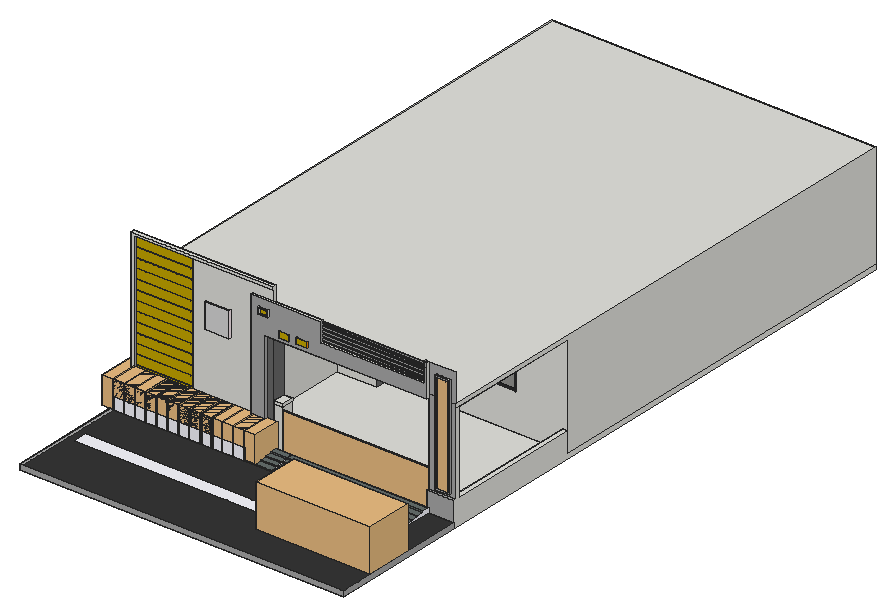
# SketchUp Ruby script. Lengths in inches.
U = 1.inch
M = Sketchup.active_model
def pt(a) = Geom::Point3d.new(a.map { |v| v * U })
def face(e, loops, mat)
  f = e.add_face(loops[0].map { |a| pt(a) })
  loops[1..].each { |l| e.add_face(l.map { |a| pt(a) }).erase! }
  f.material = f.back_material = mat if mat
  f
end
# faces: each face lists its corners as indices into pts; further lists are holes
def faces(e, pts, list, mat = nil) = list.each { |f| face(e, (f[0].is_a?(Array) ? f : [f]).map { |l| l.map { |i| pts[i] } }, mat) }
# xy, xz, yz: faces in a plane at the given z, y or x. An outline is a flat list of corners, or four numbers for a rectangle; further outlines are holes
def ring(l) = l.size == 4 ? [[l[0], l[1]], [l[2], l[1]], [l[2], l[3]], [l[0], l[3]]] : l.each_slice(2).to_a
def flat(e, list, mat, &to3) = list.each { |f| face(e, (f[0].is_a?(Array) ? f : [f]).map { |l| ring(l).map { |u, v| to3.(u, v) } }, mat) }
def xy(e, z, list, mat = nil) = flat(e, list, mat) { |x, y| [x, y, z] }
def xz(e, y, list, mat = nil) = flat(e, list, mat) { |x, z| [x, y, z] }
def yz(e, x, list, mat = nil) = flat(e, list, mat) { |y, z| [x, y, z] }
def lines(e, pts, list) = list.each { |a, b| e.add_line(pt(pts[a]), pt(pts[b])) }
# prism: a flat outline (further loops are holes) pulled along v
def prism(e, loops, v, mat = nil)
  f = face(e, loops, mat); d = Geom::Vector3d.new(v.map { |x| x * U })
  f.pushpull(f.normal.samedirection?(d) ? d.length : -d.length)
end
def box(e, o, s, mat = nil) = prism(e, [[o, [o[0] + s[0], o[1], o[2]], [o[0] + s[0], o[1] + s[1], o[2]], [o[0], o[1] + s[1], o[2]]]], [0, 0, s[2]], mat)
def at(x, y, z, deg = 0) = Geom::Transformation.translation(pt([x, y, z])) * Geom::Transformation.rotation(ORIGIN, Z_AXIS, deg.degrees)
def axes(o, x, y, z) = Geom::Transformation.new([*x, 0, *y, 0, *z, 0, *pt(o).to_a, 1])
def part(name) = M.definitions.add(name)
# library, detail: a bought-in or finely detailed component or shape, given as its bounding box
def library(name, o, s) = part(name).tap { |d| box(d.entities, o, s) }
def detail(e, o, s) = box(e.add_group.entities, o, s)
def put(e, d, t, mat = nil) = e.add_instance(d, t).tap { |i| i.material = mat if mat }
def group(e, t, mat = nil) = e.add_group.tap { |g| g.transformation = t; g.material = mat if mat }.entities
root = M.entities
M.materials.add("Glass_Tinted_Gray").color = [0, 0, 0]
M.materials["Glass_Tinted_Gray"].alpha = 0.125
M.materials.add("Shane").color = [124, 51, 43]
M.materials.add("[0008_LavenderBlush]").color = [255, 240, 245]
M.materials.add("[0019_Crimson]").color = [215, 215, 215]
M.materials.add("[0039_DarkOrange]").color = [255, 140, 0]
M.materials.add("[0046_Gold]").color = [198, 167, 0]
M.materials.add("[0117_GhostWhite]").color = [248, 248, 255]
M.materials.add("[0132_LightGray]").color = [169, 169, 169]
M.materials.add("[0134_DimGray]").color = [105, 105, 105]
M.materials.add("[0135_DarkGray]").color = [81, 81, 81]
M.materials.add("[Mirror 02]").color = [229, 229, 229]
M.materials.add("[Slate Light Tile]").color = [54, 54, 54]
M.materials.add("[Slate]").color = [102, 110, 108]
M.materials.add("[Terrazzo Light Blue]").color = [196, 214, 227]
c1 = part("door 15\#1")
xy(c1.entities,0,[[0,0,0,6,2.34,6,2.34,4,33.41,4,33.41,6,36.21,6,36.21,0,33.4,0,33.4,2,3.22,2,3.22,0]],"Shane")
xy(c1.entities,78.49,[[3.22,0,33.4,2]],"Shane")
xy(c1.entities,78.6875,[[2.34,4,33.41,6]],"Shane")
xy(c1.entities,80.63,[[0,0,36.21,6]],"Shane")
xz(c1.entities,0,[[0,0,3.22,0,3.22,78.49,33.4,78.49,33.4,0,36.21,0,36.21,80.63,0,80.63]],"Shane")
xz(c1.entities,2,[[3.22,0,33.4,78.49]],"Shane")
xz(c1.entities,4,[[2.34,0,33.41,78.6875]],"Shane")
xz(c1.entities,6,[[0,0,0,80.63,36.21,80.63,36.21,0,33.41,0,33.41,78.6875,2.34,78.6875,2.34,0]],"Shane")
yz(c1.entities,0,[[0,0,6,80.63]],"Shane")
yz(c1.entities,2.34,[[4,0,6,78.6875]],"Shane")
yz(c1.entities,3.22,[[0,0,2,78.49]],"Shane")
yz(c1.entities,33.4,[[0,0,2,78.49]],"Shane")
yz(c1.entities,33.41,[[4,0,6,78.6875]],"Shane")
yz(c1.entities,36.21,[[0,0,6,80.63]],"Shane")
c2 = part("PENTEK_RP Fineline 50S_Sliding_DoorCase_E1")
box(c2.entities,[0,0,0],[1.51,3.66,99.27],"[0135_DarkGray]")
c3 = part("PENTEK_RP Fineline 50S_SlidingDooe_Case_E2")
box(c3.entities,[0,0,0],[96.25,3.66,1.51],"[0135_DarkGray]")
c4 = part("pentek_RP Fineline 50S_SlidingDoor_Case")
put(c4.entities,c2,at(97.76,0,0))
put(c4.entities,c3,at(1.51,0,0))
put(c4.entities,c2,at(0,0,0))
put(c4.entities,c3,at(1.51,0,97.76))
c5 = part("PENTEK_RP Fineline 50S_SlidingDoor_GlazingBead_2")
box(c5.entities,[0,0,0],[0.56,0.59,94.39],"[0135_DarkGray]")
c6 = part("PENTEK_RP Fineline 50S_SlidingDoor_Glass")
box(c6.entities,[0,0,0],[46.58,0.16,94.39],"Glass_Tinted_Gray")
c7 = part("PENTEK_RP Fineline 50S_SlidingDoor_GlazingBead")
box(c7.entities,[0,0,0],[45.47,0.59,0.56],"[0135_DarkGray]")
c8 = part("PENTEK_RP Fineline 50S_SlidingDoor_Leaf_E1")
xy(c8.entities,0,[[0,0,0.93,1.97],[0.93,1.57,1.49,1.97]],"[0135_DarkGray]")
xy(c8.entities,96.25,[[0,0,0.93,0,0.93,1.57,1.49,1.57,1.49,1.97,0,1.97]],"[0135_DarkGray]")
xz(c8.entities,0,[[0,0,0.93,96.25]],"[0135_DarkGray]")
xz(c8.entities,1.57,[[0.93,0,1.49,95.32],[0.93,95.32,1.49,96.25]],"[0135_DarkGray]")
xz(c8.entities,1.97,[[0,0,1.49,96.25]],"[0135_DarkGray]")
yz(c8.entities,0,[[0,0,1.97,96.25]],"[0135_DarkGray]")
yz(c8.entities,0.93,[[0,0,1.57,0.93],[0,0.93,1.57,95.32],[0,95.32,1.57,96.25]],"[0135_DarkGray]")
yz(c8.entities,1.49,[[1.57,0,1.97,95.32],[1.57,95.32,1.97,96.25]],"[0135_DarkGray]")
c9 = part("PENTEK_RP Fineline 50S_SlidingDoor_Leaf_E2")
xy(c9.entities,0,[[0,0,0,1.57,0.56,1.57,0.56,1.97,46.02,1.97,46.02,1.57,46.58,1.57,46.58,0]],"[0135_DarkGray]")
xy(c9.entities,0.93,[[0,0,46.58,1.57]],"[0135_DarkGray]")
xy(c9.entities,1.49,[[0.56,1.57,46.02,1.97]],"[0135_DarkGray]")
xz(c9.entities,0,[[0,0,46.58,0.93]],"[0135_DarkGray]")
xz(c9.entities,1.57,[[0,0,0.56,0.93],[46.02,0,46.58,0.93],[0.56,0.93,46.02,1.49]],"[0135_DarkGray]")
xz(c9.entities,1.97,[[0.56,0,46.02,1.49]],"[0135_DarkGray]")
yz(c9.entities,0,[[0,0,1.57,0.93]],"[0135_DarkGray]")
yz(c9.entities,0.56,[[1.57,0,1.97,0.93],[1.57,0.93,1.97,1.49]],"[0135_DarkGray]")
yz(c9.entities,46.02,[[1.57,0,1.97,0.93],[1.57,0.93,1.97,1.49]],"[0135_DarkGray]")
yz(c9.entities,46.58,[[0,0,1.57,0.93]],"[0135_DarkGray]")
c10 = part("PENTEK_RP Fineline S_SlidingDoor_Leaf1")
put(c10.entities,c5,at(0.93,0,0.93))
put(c10.entities,c5,at(46.96,0,0.93))
put(c10.entities,c6,at(1.49,1.42,0.93))
put(c10.entities,c7,at(1.49,0,0.93))
put(c10.entities,c6,at(1.49,0.59,0.93),"[Terrazzo Light Blue]")
put(c10.entities,c8,at(0,0,0))
put(c10.entities,c8,axes([48.44,0,0],[-1,0,0],[0,1,0],[0,0,1]))
put(c10.entities,c9,axes([0.93,0,96.25],[1,0,0],[0,1,0],[0,0,-1]))
put(c10.entities,c9,at(0.93,0,0))
put(c10.entities,c7,at(1.49,0,94.77))
c11 = part("PENTEK_RP Fineline 50S_SlidingDoor_Leaf2")
put(c11.entities,c6,at(1.49,1.42,0.93))
put(c11.entities,c7,at(1.49,0,94.77))
put(c11.entities,c5,at(46.96,0,0.93))
put(c11.entities,c6,at(1.49,0.59,0.93),"[Mirror 02]")
put(c11.entities,c5,at(0.93,0,0.93))
put(c11.entities,c8,at(0,0,0))
put(c11.entities,c8,axes([48.44,0,0],[-1,0,0],[0,1,0],[0,0,1]))
put(c11.entities,c7,at(1.49,0,0.93))
put(c11.entities,c9,axes([0.93,0,96.25],[1,0,0],[0,1,0],[0,0,-1]))
put(c11.entities,c9,at(0.93,0,0))
c12 = part("PENTEK - Slimmest Steel Sliding Door / Window\#1")
put(c12.entities,c4,at(0,-1.88,-0.09))
put(c12.entities,c10,at(1.51,-2.27,1.42))
put(c12.entities,c11,at(49.32,-0.3,1.42))
c13 = library("new block.dwg",[0,0,0],[18.5,26.77,0.5])
c14 = library("Modern Gate 1",[0,0,0],[118.11,1.97,78.74])
c15 = library("Toyota Hilux",[0,0,0],[260.73,623.23,228.58])
c16 = part("car")
put(c16.entities,c15,axes([0,623.33,0.01],[1,0,0],[0,-1,0],[0,0,1]))
c17 = library("Palm",[82.2,-9.29,-2.36],[51.18,55.77,65.42])
c18 = library("Pinch Pot",[-27.95,-27.95,0],[55.9,55.9,47.42])
c19 = part("Potted palm")
put(c19.entities,c17,axes([3796.42,-10488.37,43.97],[0,116.51338,0],[-116.51338,0,0],[0,0,116.51338]))
put(c19.entities,c18,axes([1647.67,1801.1875,0],[0,30.58476,0],[-30.58476,0,0],[0,0,45.1095]))
c20 = library("Dome Light",[-12,-12,0],[24,24,12])
xy(root,-6,[[0,158.125,369.9375,761.125]])
xy(root,-6,[[0,0,369.9375,158.125]],"[0132_LightGray]")
xy(root,0,[[161.72,158.125,338.91,158.125,338.91,164.5,363.9375,164.5,363.9375,321.3125,217.72,321.3125,217.72,365,170.41,365,170.41,321.3125,161.72,321.3125,161.72,307.89,116.03,307.89,116.03,174.55,161.72,174.55,161.72,174.375,171.53,174.375,171.53,161.125,161.72,161.125],[0,159.125,4,159.125,4,160.625,68.79,160.625,68.79,161.125,161.72,161.125,161.72,174.55,116.03,174.55,116.03,307.89,161.72,307.89,161.72,321.3125,170.41,321.3125,170.41,365,217.72,365,217.72,321.3125,369.9375,321.3125,369.9375,761.125,0,761.125]])
xy(root,0,[[12.52,63.38,351.27,78.51],[184.6875,129.125,340.6875,158.125],[6.76,131.88,151.49,155.37]],"[0117_GhostWhite]")
xy(root,0,[[0,0,4,129.125],[0,129.125,4,158.125],[154.25,129.125,184.6875,158.125],[0,158.125,4,159.125],[4,158.125,68.79,160.625],
  [68.79,158.125,137.31,161.125],[137.31,158.125,153.78,161.125],[153.78,158.125,161.72,161.125]],"[0132_LightGray]")
xy(root,0,[[[4,0,369.9375,0,369.9375,158.125,340.6875,158.125,340.6875,129.125,4,129.125],[12.52,63.38,351.27,78.51]]],"[Slate Light Tile]")
xy(root,1.25,[[154.25,129.125,184.6875,136.375],[184.6875,129.125,340.6875,136.375]],"[Slate]")
xy(root,2.375,[[154.25,136.375,184.6875,143.625],[184.6875,136.375,340.6875,143.625]],"[Slate]")
xy(root,3.5,[[154.25,143.625,184.6875,150.875],[184.6875,143.625,340.6875,150.875]],"[Slate]")
xy(root,4.875,[[154.25,150.875,184.6875,158.125],[184.6875,150.875,340.6875,158.125]],"[Slate]")
xy(root,10.38,[[4,160.625,68.79,161.125]])
xy(root,10.98,[[4,160.625,68.79,161.125]])
xy(root,13.4375,[[[4,129.125,154.25,158.125],[6.76,131.88,151.49,155.37]]],"[0117_GhostWhite]")
xy(root,21.37,[[4,160.625,68.79,161.125]])
xy(root,21.97,[[4,160.625,68.79,161.125]])
xy(root,22.8125,[[363.9375,164.5,369.9375,321.3125]])
xy(root,22.8125,[[338.91,158.125,369.9375,161.125]],"[0132_LightGray]")
xy(root,25.96,[[347.38,158.75,364.45,161.125]])
xy(root,28.16,[[349.58,158.75,362.25,161.125]])
xy(root,32.35,[[4,160.625,68.79,161.125]])
xy(root,32.95,[[4,160.625,68.79,161.125]])
xy(root,41.52,[[244.46,321.3125,309.58,347.625]])
xy(root,43.33,[[4,160.625,68.79,161.125]])
xy(root,43.93,[[4,160.625,68.79,161.125]])
xy(root,48,[[161.72,160.625,172.03,161.125],[161.72,161.125,171.53,174.375],[171.53,161.125,172.03,174.55],[161.72,174.375,171.53,174.55]])
xy(root,51,[[161.72,160.625,172.03,174.55]])
xy(root,54.32,[[4,160.625,68.79,161.125]])
xy(root,54.92,[[4,160.625,68.79,161.125]])
xy(root,65.3,[[4,160.625,68.79,161.125]])
xy(root,65.9,[[4,160.625,68.79,161.125]])
xy(root,76.28,[[4,160.625,68.79,161.125]])
xy(root,76.88,[[4,160.625,68.79,161.125]])
xy(root,87.27,[[4,160.625,68.79,161.125]])
xy(root,87.87,[[4,160.625,68.79,161.125]])
xy(root,93.58,[[244.46,321.3125,309.58,347.625]])
xy(root,94.375,[[170.41,321.3125,217.72,365]])
xy(root,97.96,[[84.13,158.5625,111.94,161.125]],"[0008_LavenderBlush]")
xy(root,98.25,[[4,160.625,68.79,161.125]])
xy(root,98.85,[[4,160.625,68.79,161.125]])
xy(root,102.58,[[116.03,174.55,161.72,307.89]])
xy(root,109.23,[[4,160.625,68.79,161.125]])
xy(root,109.83,[[4,160.625,68.79,161.125]])
xy(root,116,[[161.72,161.125,161.72,321.3125,271.17,321.3125,367.86,164.5,338.91,164.5,338.91,161.125],[369.9375,161.125,367.86,164.5,369.9375,164.5],[367.86,164.5,271.17,321.3125,369.9375,321.3125,369.9375,164.5]])
xy(root,116,[[153.78,158.125,338.91,161.125]],"[0132_LightGray]")
xy(root,119.85,[[170.43,157.43,181.45,158.125]],"[0039_DarkOrange]")
xy(root,120,[[161.72,161.125,369.9375,161.125,369.9375,761.125,0,761.125,0,163.25,161.72,163.25]])
xy(root,120.17,[[189.76,157.43,202.51,158.125]],"[0039_DarkOrange]")
xy(root,120.22,[[4,160.625,68.79,161.125]])
xy(root,120.82,[[4,160.625,68.79,161.125]])
xy(root,125.77,[[84.13,158.5625,111.94,161.125]],"[0008_LavenderBlush]")
xy(root,126.67,[[170.43,157.43,181.45,158.125]],"[0039_DarkOrange]")
xy(root,126.74,[[189.76,157.43,202.51,158.125]],"[0039_DarkOrange]")
xy(root,131.0625,[[217.73,158.125,335.04,161.125]])
xy(root,131.2,[[4,160.625,68.79,161.125]])
xy(root,131.8,[[4,160.625,68.79,161.125]])
xy(root,133.74,[[217.73,158.86,335.73,160.42]])
xy(root,135.3,[[217.73,158.86,335.73,160.42]],"[0132_LightGray]")
xy(root,136.46,[[146.93,156.6875,158.46,158.125]])
xy(root,137.27,[[147.74,156.6875,157.65,158.125]])
xy(root,137.93,[[217.73,158.86,336.85,160.42]])
xy(root,139.49,[[217.73,158.86,336.85,160.42]],"[0132_LightGray]")
xy(root,141.33,[[349.58,158.75,362.25,161.125]])
xy(root,142.11,[[217.73,158.86,337.16,160.42]])
xy(root,142.18,[[4,160.625,68.79,161.125]])
xy(root,142.78,[[147.74,156.6875,157.65,158.125],[4,160.625,68.79,161.125]])
xy(root,143.53,[[347.38,158.75,364.45,161.125]])
xy(root,143.59,[[146.93,156.6875,158.46,158.125]])
xy(root,143.68,[[217.73,158.86,337.16,160.42]],"[0132_LightGray]")
xy(root,146.3,[[217.73,158.86,336.54,160.42]])
xy(root,147.86,[[217.73,158.86,336.54,160.42]])
xy(root,150.49,[[217.73,158.86,338.66,160.42]])
xy(root,152.05,[[217.73,158.86,338.66,160.42]])
xy(root,152.8125,[[137.31,158.125,217.73,161.125],[335.04,158.125,338.91,161.125]])
xy(root,153.17,[[4,160.625,68.79,161.125]])
xy(root,153.77,[[4,160.625,68.79,161.125]])
xy(root,164.75,[[4,159.125,4,160.625,68.79,160.625,68.79,161.125,161.72,161.125,161.72,159.125]])
xy(root,168,[[0,159.125,161.72,163.25]])
xz(root,0,[[0,-6,369.9375,0]],"[0132_LightGray]")
xz(root,129.125,[[4,0,154.25,13.4375]],"[0117_GhostWhite]")
xz(root,129.125,[[154.25,0,184.6875,1.25]],"[0132_LightGray]")
xz(root,129.125,[[184.6875,0,340.6875,1.25]],"[Slate]")
xz(root,131.88,[[6.76,0,151.49,13.4375]],"[0117_GhostWhite]")
xz(root,136.375,[[154.25,1.25,184.6875,2.375],[184.6875,1.25,340.6875,2.375]],"[Slate]")
xz(root,143.625,[[154.25,2.375,184.6875,3.5],[184.6875,2.375,340.6875,3.5]],"[Slate]")
xz(root,150.875,[[154.25,3.5,184.6875,4.875],[184.6875,3.5,340.6875,4.875]],"[Slate]")
xz(root,155.37,[[6.76,0,151.49,13.4375]],"[0117_GhostWhite]")
xz(root,156.6875,[[[146.93,136.46,158.46,143.59],[147.74,137.27,157.65,142.78]]])
xz(root,157.43,[[170.43,119.85,181.45,126.67],[189.76,120.17,202.51,126.74]],"[0046_Gold]")
xz(root,158.125,[[147.74,137.27,157.65,142.78]],"[0046_Gold]")
xz(root,158.125,[[184.6875,0,338.91,4.875]],"[0117_GhostWhite]")
xz(root,158.125,[[0,-6,369.9375,0],[4,0,68.79,13.4375],[68.79,0,137.31,13.4375],[137.31,0,153.78,13.4375],[153.78,0,154.25,13.4375],
  [154.25,0,184.6875,4.875],[338.91,0,340.6875,4.875],[340.6875,0,369.9375,0,369.9375,22.8125,338.91,22.8125,338.91,4.875,340.6875,4.875],[[137.31,13.4375,153.78,13.4375,153.78,116,338.91,116,338.91,152.8125,335.04,152.8125,335.04,131.0625,217.73,131.0625,217.73,152.8125,137.31,152.8125],[189.76,120.17,202.51,126.74],[146.93,136.46,158.46,143.59],[170.43,119.85,181.45,126.67]]],"[0132_LightGray]")
xz(root,158.5625,[[84.13,97.96,111.94,125.77]],"[0019_Crimson]")
xz(root,158.75,[[[347.38,25.96,364.45,143.53],[349.58,28.16,362.25,141.33]]],"[0132_LightGray]")
xz(root,158.86,[[217.73,133.74,335.73,135.3],[217.73,137.93,336.85,139.49],[217.73,142.11,337.16,143.68],[217.73,146.3,336.54,147.86],[217.73,150.49,338.66,152.05]],"[0132_LightGray]")
xz(root,159.125,[[0,0,4,0,4,164.75,161.72,164.75,161.72,168,0,168]])
xz(root,160.42,[[217.73,133.74,335.73,135.3],[217.73,137.93,336.85,139.49],[217.73,142.11,337.16,143.68],[217.73,146.3,336.54,147.86],[217.73,150.49,338.66,152.05]],"[0132_LightGray]")
xz(root,160.625,[[161.72,48,172.03,51]])
xz(root,160.625,[[4,0,68.79,10.38],[4,10.98,68.79,21.37],[4,21.97,68.79,32.35],[4,32.95,68.79,43.33],[4,43.93,68.79,54.32],
  [4,54.92,68.79,65.3],[4,65.9,68.79,76.28],[4,76.88,68.79,87.27],[4,87.87,68.79,98.25],[4,98.85,68.79,109.23],
  [4,109.83,68.79,120.22],[4,120.82,68.79,131.2],[4,131.8,68.79,142.18],[4,142.78,68.79,153.17],[4,153.77,68.79,164.75]],"[0046_Gold]")
xz(root,161.125,[[[68.79,0,137.31,0,137.31,152.8125,161.72,152.8125,161.72,164.75,68.79,164.75],[84.13,97.96,111.94,125.77]],[161.72,0,171.53,48],[347.38,25.96,364.45,25.96,364.45,120,362.25,120,362.25,28.16,349.58,28.16,349.58,120,347.38,120],[347.38,120,349.58,120,349.58,141.33,362.25,141.33,362.25,120,364.45,120,364.45,143.53,347.38,143.53]])
xz(root,161.125,[[137.31,0,137.31,120,338.91,120,338.91,116,153.78,116,153.78,0],[4,10.38,68.79,10.98],[4,21.37,68.79,21.97],[338.91,22.8125,369.9375,22.8125,369.9375,120,364.45,120,364.45,25.96,347.38,25.96,347.38,120,338.91,120],[349.58,28.16,362.25,120],
  [4,32.35,68.79,32.95],[4,43.33,68.79,43.93],[4,54.32,68.79,54.92],[4,65.3,68.79,65.9],[4,76.28,68.79,76.88],
  [4,87.27,68.79,87.87],[4,98.25,68.79,98.85],[4,109.23,68.79,109.83],[137.31,120,161.72,152.8125],[161.72,120,161.72,152.8125,217.73,152.8125,217.73,131.0625,335.04,131.0625,335.04,152.8125,338.91,152.8125,338.91,120],
  [338.91,120,347.38,120,347.38,143.53,364.45,143.53,364.45,120,369.9375,120,369.9375,152.8125,338.91,152.8125],[349.58,120,362.25,141.33],[4,120.22,68.79,120.82],[4,131.2,68.79,131.8],[4,142.18,68.79,142.78],
  [4,153.17,68.79,153.77]],"[0132_LightGray]")
xz(root,161.125,[[153.78,0,161.72,116]],"[0134_DimGray]")
xz(root,163.25,[[0,120,161.72,168]])
xz(root,164.5,[[338.91,0,338.91,116,369.9375,116,369.9375,22.8125,363.9375,22.8125,363.9375,0]])
xz(root,174.375,[[161.72,0,171.53,48]])
xz(root,174.55,[[116.03,0,161.72,102.58],[161.72,48,172.03,51]])
xz(root,307.89,[[116.03,0,161.72,102.58]])
xz(root,321.3125,[[[161.72,0,170.41,0,170.41,94.375,217.72,94.375,217.72,0,363.9375,0,363.9375,22.8125,369.9375,22.8125,369.9375,116,161.72,116],[244.46,41.52,309.58,93.58]],[363.9375,0,369.9375,22.8125]])
xz(root,347.625,[[244.46,41.52,309.58,93.58]])
xz(root,365,[[170.41,0,217.72,94.375]])
xz(root,761.125,[[0,-6,369.9375,0],[0,0,369.9375,120]])
yz(root,0,[[158.125,-6,761.125,0],[159.125,0,159.125,168,163.25,168,163.25,120,761.125,120,761.125,0]])
yz(root,0,[[0,-6,158.125,0]],"[0132_LightGray]")
yz(root,4,[[129.125,0,158.125,13.4375]],"[0117_GhostWhite]")
yz(root,4,[[159.125,0,160.625,0,160.625,10.38,161.125,10.38,161.125,10.98,160.625,10.98,160.625,21.37,161.125,21.37,161.125,21.97,160.625,21.97,160.625,32.35,161.125,32.35,161.125,32.95,160.625,32.95,160.625,43.33,161.125,43.33,161.125,43.93,160.625,43.93,160.625,54.32,161.125,54.32,161.125,54.92,160.625,54.92,160.625,65.3,161.125,65.3,161.125,65.9,160.625,65.9,160.625,76.28,161.125,76.28,161.125,76.88,160.625,76.88,160.625,87.27,161.125,87.27,161.125,87.87,160.625,87.87,160.625,98.25,161.125,98.25,161.125,98.85,160.625,98.85,160.625,109.23,161.125,109.23,161.125,109.83,160.625,109.83,160.625,120.22,161.125,120.22,161.125,120.82,160.625,120.82,160.625,131.2,161.125,131.2,161.125,131.8,160.625,131.8,160.625,142.18,161.125,142.18,161.125,142.78,160.625,142.78,160.625,153.17,161.125,153.17,161.125,153.77,160.625,153.77,160.625,164.75,159.125,164.75]],"[0132_LightGray]")
yz(root,6.76,[[131.88,0,155.37,13.4375]],"[0132_LightGray]")
yz(root,68.79,[[160.625,0,161.125,10.38],[160.625,10.98,161.125,21.37],[160.625,21.97,161.125,32.35],[160.625,32.95,161.125,43.33],[160.625,43.93,161.125,54.32],
  [160.625,54.92,161.125,65.3],[160.625,65.9,161.125,76.28],[160.625,76.88,161.125,87.27],[160.625,87.87,161.125,98.25],[160.625,98.85,161.125,109.23],
  [160.625,109.83,161.125,120.22],[160.625,120.82,161.125,131.2],[160.625,131.8,161.125,142.18],[160.625,142.78,161.125,153.17],[160.625,153.77,161.125,164.75]])
yz(root,84.13,[[158.5625,97.96,161.125,125.77]],"[0008_LavenderBlush]")
yz(root,111.94,[[158.5625,97.96,161.125,125.77]],"[0008_LavenderBlush]")
yz(root,116.03,[[174.55,0,307.89,102.58]])
yz(root,137.31,[[158.125,0,161.125,152.8125]])
yz(root,146.93,[[156.6875,136.46,158.125,143.59]])
yz(root,147.74,[[156.6875,137.27,158.125,142.78]])
yz(root,151.49,[[131.88,0,155.37,13.4375]],"[0117_GhostWhite]")
yz(root,153.78,[[158.125,0,161.125,116]],"[0132_LightGray]")
yz(root,154.25,[[129.125,0,129.125,1.25,136.375,1.25,136.375,2.375,143.625,2.375,143.625,3.5,150.875,3.5,150.875,4.875,158.125,4.875,158.125,0],[129.125,1.25,136.375,13.4375],[136.375,2.375,143.625,13.4375],[143.625,3.5,150.875,13.4375],[150.875,4.875,158.125,13.4375]],"[0132_LightGray]")
yz(root,157.65,[[156.6875,137.27,158.125,142.78]])
yz(root,158.46,[[156.6875,136.46,158.125,143.59]])
yz(root,161.72,[[161.125,0,174.375,48],[174.375,0,174.55,48],[160.625,48,161.125,51],[161.125,48,174.55,51],[161.125,120,163.25,120,163.25,168,159.125,168,159.125,164.75,161.125,164.75]])
yz(root,161.72,[[307.89,0,321.3125,0,321.3125,116,161.125,116,161.125,51,174.55,51,174.55,102.58,307.89,102.58]],"[0134_DimGray]")
yz(root,170.41,[[321.3125,0,365,94.375]])
yz(root,170.43,[[157.43,119.85,158.125,126.67]],"[0039_DarkOrange]")
yz(root,171.53,[[161.125,0,174.375,48]])
yz(root,172.03,[[160.625,48,174.55,51]])
yz(root,181.45,[[157.43,119.85,158.125,126.67]],"[0039_DarkOrange]")
yz(root,184.6875,[[129.125,0,129.125,1.25,136.375,1.25,136.375,2.375,143.625,2.375,143.625,3.5,150.875,3.5,150.875,4.875,158.125,4.875,158.125,0]],"[0117_GhostWhite]")
yz(root,189.76,[[157.43,120.17,158.125,126.74]],"[0039_DarkOrange]")
yz(root,202.51,[[157.43,120.17,158.125,126.74]],"[0039_DarkOrange]")
yz(root,217.72,[[321.3125,0,365,94.375]])
yz(root,217.73,[[[158.125,131.0625,161.125,152.8125],[158.86,133.74,160.42,135.3],[158.86,137.93,160.42,139.49],[158.86,142.11,160.42,143.68],[158.86,146.3,160.42,147.86],[158.86,150.49,160.42,152.05]]],"[0132_LightGray]")
yz(root,244.46,[[321.3125,41.52,347.625,93.58]])
yz(root,309.58,[[321.3125,41.52,347.625,93.58]])
yz(root,335.04,[[158.125,131.0625,161.125,152.8125]],"[0132_LightGray]")
yz(root,335.73,[[158.86,133.74,160.42,135.3]])
yz(root,336.54,[[158.86,146.3,160.42,147.86]])
yz(root,336.85,[[158.86,137.93,160.42,139.49]])
yz(root,337.16,[[158.86,142.11,160.42,143.68]])
yz(root,338.66,[[158.86,150.49,160.42,152.05]])
yz(root,338.91,[[161.125,0,164.5,116],[158.125,116,161.125,152.8125]])
yz(root,338.91,[[158.125,0,161.125,22.8125]],"[0132_LightGray]")
yz(root,340.6875,[[129.125,0,158.125,0,158.125,4.875,150.875,4.875,150.875,3.5,143.625,3.5,143.625,2.375,136.375,2.375,136.375,1.25,129.125,1.25]],"[0117_GhostWhite]")
yz(root,347.38,[[158.75,25.96,161.125,143.53]])
yz(root,349.58,[[158.75,28.16,161.125,141.33]],"[0132_LightGray]")
yz(root,362.25,[[158.75,28.16,161.125,141.33]])
yz(root,363.9375,[[164.5,0,321.3125,22.8125]])
yz(root,364.45,[[158.75,25.96,161.125,143.53]],"[0132_LightGray]")
yz(root,369.9375,[[158.125,-6,761.125,-6,761.125,0,321.3125,0,321.3125,22.8125,164.5,22.8125,164.5,116,161.125,116,161.125,22.8125,158.125,22.8125],[321.3125,0,761.125,0,761.125,120,161.125,120,161.125,116,321.3125,116]])
yz(root,369.9375,[[0,-6,158.125,0]],"[0132_LightGray]")
p = [[271.17,321.3125,116],[0,761.125,116],[0,161.125,120],[0,163.25,120],[68.79,161.125,120],[-943.1875,836.75,0],
  [-942.59,836.75,0],[-229.54,-1013.375,-973.6],[-229.54,-1012.78,-973.6],[1554.09,-733.33,0],[1554.6875,-733.33,0]]
lines(root,p,[[0,1],[2,3],[4,2],[5,6],[7,8],[9,10]])
put(root,c1,axes([170.41,321.3125,0],[1.30679,0,0],[0,1,0],[0,0,1.17049]))
put(root,c12,axes([243.55,322.47,41.48],[0.6652,0,0],[0,0.35,0],[0,0,0.52536]))
put(root,c13,axes([349.58,159.03,28.16],[0.6893,0,0],[0,0,4.22746],[0,-0.61,0]),"[0132_LightGray]")
put(root,c14,axes([171.53,161.125,0],[1.41713,0,0],[0,1,0],[0,0,0.5559]),"[0117_GhostWhite]")
put(root,c16,axes([238.6,93.16,0],[0,-0.21,0],[0.21,0,0],[0,0,0.21]))
put(root,c19,axes([129.13,135.96,0.9375],[0.0075,0,0],[0,0.0075,0],[0,0,0.00405]))
put(root,c19,axes([116.47,135.96,0.9375],[0.0075,0,0],[0,0.0075,0],[0,0,0.00405]))
put(root,c19,axes([103.81,135.96,0.9375],[0.0075,0,0],[0,0.0075,0],[0,0,0.00405]))
put(root,c19,axes([91.14,135.96,0.9375],[0.0075,0,0],[0,0.0075,0],[0,0,0.00405]))
put(root,c19,axes([78.48,135.96,0.9375],[0.0075,0,0],[0,0.0075,0],[0,0,0.00405]))
put(root,c19,axes([65.82,135.96,0.9375],[0.0075,0,0],[0,0.0075,0],[0,0,0.00405]))
put(root,c19,axes([53.16,135.96,0.9375],[0.0075,0,0],[0,0.0075,0],[0,0,0.00405]))
put(root,c19,axes([40.49,135.96,0.9375],[0.0075,0,0],[0,0.0075,0],[0,0,0.00405]))
put(root,c19,axes([27.83,135.96,0.9375],[0.0075,0,0],[0,0.0075,0],[0,0,0.00405]))
put(root,c19,axes([15.17,135.96,0.9375],[0.0075,0,0],[0,0.0075,0],[0,0,0.00405]))
put(root,c19,axes([2.51,135.96,0.9375],[0.0075,0,0],[0,0.0075,0],[0,0,0.00405]))
put(root,c20,at(-28.875,303.08,0))
